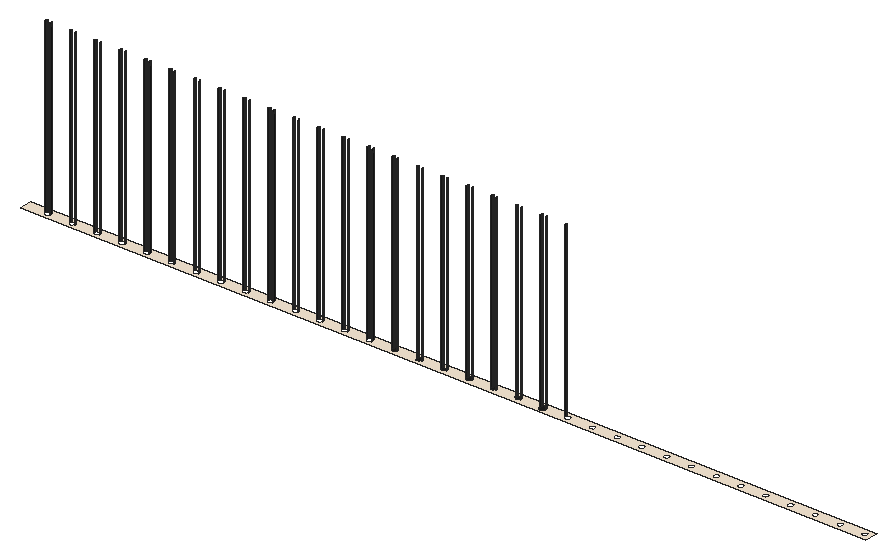
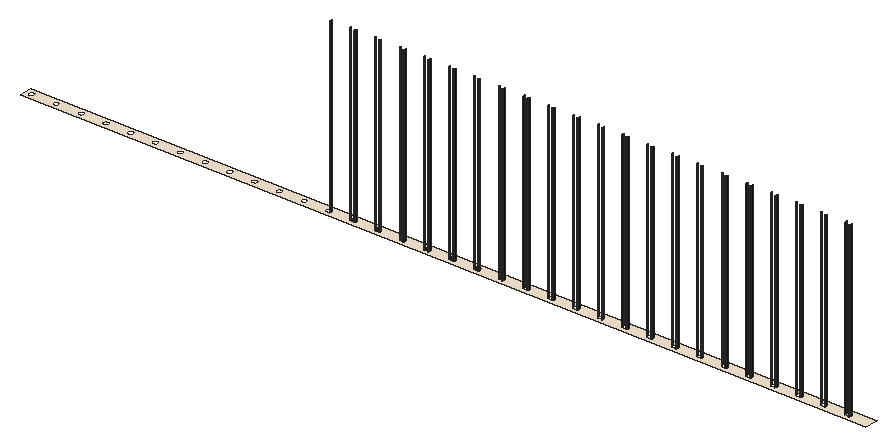
# SketchUp Ruby script. Lengths in inches.
U = 1.inch
M = Sketchup.active_model
def pt(a) = Geom::Point3d.new(a.map { |v| v * U })
def face(e, loops, mat)
  f = e.add_face(loops[0].map { |a| pt(a) })
  loops[1..].each { |l| e.add_face(l.map { |a| pt(a) }).erase! }
  f.material = f.back_material = mat if mat
  f
end
# faces: each face lists its corners as indices into pts; further lists are holes
def faces(e, pts, list, mat = nil) = list.each { |f| face(e, (f[0].is_a?(Array) ? f : [f]).map { |l| l.map { |i| pts[i] } }, mat) }
# xy, xz, yz: faces in a plane at the given z, y or x. An outline is a flat list of corners, or four numbers for a rectangle; further outlines are holes
def ring(l) = l.size == 4 ? [[l[0], l[1]], [l[2], l[1]], [l[2], l[3]], [l[0], l[3]]] : l.each_slice(2).to_a
def flat(e, list, mat, &to3) = list.each { |f| face(e, (f[0].is_a?(Array) ? f : [f]).map { |l| ring(l).map { |u, v| to3.(u, v) } }, mat) }
def xy(e, z, list, mat = nil) = flat(e, list, mat) { |x, y| [x, y, z] }
def xz(e, y, list, mat = nil) = flat(e, list, mat) { |x, z| [x, y, z] }
def yz(e, x, list, mat = nil) = flat(e, list, mat) { |y, z| [x, y, z] }
def lines(e, pts, list) = list.each { |a, b| e.add_line(pt(pts[a]), pt(pts[b])) }
# prism: a flat outline (further loops are holes) pulled along v
def prism(e, loops, v, mat = nil)
  f = face(e, loops, mat); d = Geom::Vector3d.new(v.map { |x| x * U })
  f.pushpull(f.normal.samedirection?(d) ? d.length : -d.length)
end
def box(e, o, s, mat = nil) = prism(e, [[o, [o[0] + s[0], o[1], o[2]], [o[0] + s[0], o[1] + s[1], o[2]], [o[0], o[1] + s[1], o[2]]]], [0, 0, s[2]], mat)
def at(x, y, z, deg = 0) = Geom::Transformation.translation(pt([x, y, z])) * Geom::Transformation.rotation(ORIGIN, Z_AXIS, deg.degrees)
def axes(o, x, y, z) = Geom::Transformation.new([*x, 0, *y, 0, *z, 0, *pt(o).to_a, 1])
def part(name) = M.definitions.add(name)
# library, detail: a bought-in or finely detailed component or shape, given as its bounding box
def library(name, o, s) = part(name).tap { |d| box(d.entities, o, s) }
def detail(e, o, s) = box(e.add_group.entities, o, s)
def put(e, d, t, mat = nil) = e.add_instance(d, t).tap { |i| i.material = mat if mat }
def group(e, t, mat = nil) = e.add_group.tap { |g| g.transformation = t; g.material = mat if mat }.entities
root = M.entities
M.materials.add("[0028_AntiqueWhite]").color = [250, 235, 215]
M.materials.add("[Color M08]").color = [30, 30, 30]
xy(root,177,[[[50.75,194.125,206.5625,196.4375],[54.79,194.68,54.65,194.71,54.52,194.79,54.42,194.89,54.35,195.02,54.31,195.16,54.31,195.31,54.34,195.45,54.42,195.58,54.52,195.68,54.65,195.75,54.79,195.79,54.9375,195.79,55.08,195.75,55.21,195.68,55.31,195.58,55.38,195.45,55.42,195.31,55.42,195.16,55.38,195.02,55.3125,194.89,55.21,194.79,55.08,194.72,54.9375,194.68],[59.35,194.68,59.21,194.71,59.09,194.79,58.98,194.89,58.91,195.02,58.87,195.16,58.87,195.31,58.91,195.45,58.98,195.58,59.08,195.68,59.21,195.75,59.35,195.79,59.5,195.79,59.64,195.75,59.77,195.68,59.87,195.58,59.95,195.45,59.98,195.31,59.99,195.16,59.95,195.02,59.875,194.89,59.77,194.79,59.64,194.72,59.5,194.68],[63.92,194.68,63.78,194.71,63.65,194.79,63.54,194.89,63.47,195.02,63.43,195.16,63.43,195.31,63.47,195.45,63.54,195.58,63.65,195.68,63.77,195.75,63.92,195.79,64.0625,195.79,64.2,195.75,64.33,195.68,64.44,195.58,64.51,195.45,64.55,195.31,64.55,195.16,64.51,195.02,64.4375,194.89,64.33,194.79,64.21,194.72,64.0625,194.68],[68.48,194.68,68.34,194.71,68.21,194.79,68.11,194.89,68.03,195.02,67.99,195.16,67.99,195.31,68.03,195.45,68.11,195.58,68.21,195.68,68.34,195.75,68.48,195.79,68.625,195.79,68.77,195.75,68.89,195.68,69,195.58,69.07,195.45,69.11,195.31,69.11,195.16,69.07,195.02,69,194.89,68.9,194.79,68.77,194.72,68.625,194.68],[73.04,194.68,72.9,194.71,72.77,194.79,72.67,194.89,72.6,195.02,72.56,195.16,72.56,195.31,72.59,195.45,72.67,195.58,72.77,195.68,72.9,195.75,73.04,195.79,73.1875,195.79,73.33,195.75,73.46,195.68,73.56,195.58,73.63,195.45,73.67,195.31,73.67,195.16,73.63,195.02,73.5625,194.89,73.46,194.79,73.33,194.72,73.1875,194.68],[77.6,194.68,77.46,194.71,77.34,194.79,77.23,194.89,77.16,195.02,77.12,195.16,77.12,195.31,77.16,195.45,77.23,195.58,77.33,195.68,77.46,195.75,77.6,195.79,77.75,195.79,77.89,195.75,78.02,195.68,78.12,195.58,78.2,195.45,78.23,195.31,78.24,195.16,78.2,195.02,78.125,194.89,78.02,194.79,77.89,194.72,77.75,194.68],[82.17,194.68,82.03,194.71,81.9,194.79,81.79,194.89,81.72,195.02,81.68,195.16,81.68,195.31,81.72,195.45,81.79,195.58,81.9,195.68,82.02,195.75,82.17,195.79,82.3125,195.79,82.45,195.75,82.58,195.68,82.69,195.58,82.76,195.45,82.8,195.31,82.8,195.16,82.76,195.02,82.6875,194.89,82.58,194.79,82.46,194.72,82.3125,194.68],[86.73,194.68,86.59,194.71,86.46,194.79,86.36,194.89,86.28,195.02,86.24,195.16,86.24,195.31,86.28,195.45,86.36,195.58,86.46,195.68,86.59,195.75,86.73,195.79,86.875,195.79,87.02,195.75,87.14,195.68,87.25,195.58,87.32,195.45,87.36,195.31,87.36,195.16,87.32,195.02,87.25,194.89,87.15,194.79,87.02,194.72,86.875,194.68],[91.29,194.68,91.15,194.71,91.02,194.79,90.92,194.89,90.85,195.02,90.81,195.16,90.81,195.31,90.84,195.45,90.92,195.58,91.02,195.68,91.15,195.75,91.29,195.79,91.4375,195.79,91.58,195.75,91.71,195.68,91.81,195.58,91.88,195.45,91.92,195.31,91.92,195.16,91.88,195.02,91.8125,194.89,91.71,194.79,91.58,194.72,91.4375,194.68],[95.85,194.68,95.71,194.71,95.59,194.79,95.48,194.89,95.41,195.02,95.37,195.16,95.37,195.31,95.41,195.45,95.48,195.58,95.58,195.68,95.71,195.75,95.85,195.79,96,195.79,96.14,195.75,96.27,195.68,96.37,195.58,96.45,195.45,96.48,195.31,96.49,195.16,96.45,195.02,96.375,194.89,96.27,194.79,96.14,194.72,96,194.68],[100.42,194.68,100.28,194.71,100.15,194.79,100.04,194.89,99.97,195.02,99.93,195.16,99.93,195.31,99.97,195.45,100.04,195.58,100.15,195.68,100.27,195.75,100.42,195.79,100.5625,195.79,100.7,195.75,100.83,195.68,100.94,195.58,101.01,195.45,101.05,195.31,101.05,195.16,101.01,195.02,100.9375,194.89,100.83,194.79,100.71,194.72,100.5625,194.68],[104.98,194.68,104.84,194.71,104.71,194.79,104.61,194.89,104.53,195.02,104.49,195.16,104.49,195.31,104.53,195.45,104.61,195.58,104.71,195.68,104.84,195.75,104.98,195.79,105.125,195.79,105.27,195.75,105.39,195.68,105.5,195.58,105.57,195.45,105.61,195.31,105.61,195.16,105.57,195.02,105.5,194.89,105.4,194.79,105.27,194.72,105.125,194.68],[109.54,194.68,109.4,194.71,109.27,194.79,109.17,194.89,109.1,195.02,109.06,195.16,109.06,195.31,109.09,195.45,109.17,195.58,109.27,195.68,109.4,195.75,109.54,195.79,109.6875,195.79,109.83,195.75,109.96,195.68,110.06,195.58,110.13,195.45,110.17,195.31,110.17,195.16,110.13,195.02,110.0625,194.89,109.96,194.79,109.83,194.72,109.6875,194.68],[114.1,194.68,113.96,194.71,113.84,194.79,113.73,194.89,113.66,195.02,113.62,195.16,113.62,195.31,113.66,195.45,113.73,195.58,113.83,195.68,113.96,195.75,114.1,195.79,114.25,195.79,114.39,195.75,114.52,195.68,114.62,195.58,114.7,195.45,114.73,195.31,114.74,195.16,114.7,195.02,114.625,194.89,114.52,194.79,114.39,194.72,114.25,194.68],[118.67,194.68,118.53,194.71,118.4,194.79,118.29,194.89,118.22,195.02,118.18,195.16,118.18,195.31,118.22,195.45,118.29,195.58,118.4,195.68,118.52,195.75,118.67,195.79,118.8125,195.79,118.95,195.75,119.08,195.68,119.19,195.58,119.26,195.45,119.3,195.31,119.3,195.16,119.26,195.02,119.1875,194.89,119.08,194.79,118.96,194.72,118.8125,194.68],[123.23,194.68,123.09,194.71,122.96,194.79,122.86,194.89,122.78,195.02,122.74,195.16,122.74,195.31,122.78,195.45,122.86,195.58,122.96,195.68,123.09,195.75,123.23,195.79,123.375,195.79,123.52,195.75,123.64,195.68,123.75,195.58,123.82,195.45,123.86,195.31,123.86,195.16,123.82,195.02,123.75,194.89,123.65,194.79,123.52,194.72,123.375,194.68],[127.79,194.68,127.65,194.71,127.52,194.79,127.42,194.89,127.35,195.02,127.31,195.16,127.31,195.31,127.34,195.45,127.42,195.58,127.52,195.68,127.65,195.75,127.79,195.79,127.9375,195.79,128.08,195.75,128.21,195.68,128.31,195.58,128.38,195.45,128.42,195.31,128.42,195.16,128.38,195.02,128.3125,194.89,128.21,194.79,128.08,194.72,127.9375,194.68],[132.35,194.68,132.21,194.71,132.09,194.79,131.98,194.89,131.91,195.02,131.87,195.16,131.87,195.31,131.91,195.45,131.98,195.58,132.08,195.68,132.21,195.75,132.35,195.79,132.5,195.79,132.64,195.75,132.77,195.68,132.87,195.58,132.95,195.45,132.98,195.31,132.99,195.16,132.95,195.02,132.875,194.89,132.77,194.79,132.64,194.72,132.5,194.68],[136.92,194.68,136.78,194.71,136.65,194.79,136.54,194.89,136.47,195.02,136.43,195.16,136.43,195.31,136.47,195.45,136.54,195.58,136.65,195.68,136.77,195.75,136.92,195.79,137.0625,195.79,137.2,195.75,137.33,195.68,137.44,195.58,137.51,195.45,137.55,195.31,137.55,195.16,137.51,195.02,137.4375,194.89,137.33,194.79,137.21,194.72,137.0625,194.68],[141.48,194.68,141.34,194.71,141.21,194.79,141.11,194.89,141.03,195.02,140.99,195.16,140.99,195.31,141.03,195.45,141.11,195.58,141.21,195.68,141.34,195.75,141.48,195.79,141.625,195.79,141.77,195.75,141.89,195.68,142,195.58,142.07,195.45,142.11,195.31,142.11,195.16,142.07,195.02,142,194.89,141.9,194.79,141.77,194.72,141.625,194.68],[146.04,194.68,145.9,194.71,145.77,194.79,145.67,194.89,145.6,195.02,145.56,195.16,145.56,195.31,145.59,195.45,145.67,195.58,145.77,195.68,145.9,195.75,146.04,195.79,146.1875,195.79,146.33,195.75,146.46,195.68,146.56,195.58,146.63,195.45,146.67,195.31,146.67,195.16,146.63,195.02,146.5625,194.89,146.46,194.79,146.33,194.72,146.1875,194.68],[150.6,194.68,150.46,194.71,150.34,194.79,150.23,194.89,150.16,195.02,150.12,195.16,150.12,195.31,150.16,195.45,150.23,195.58,150.33,195.68,150.46,195.75,150.6,195.79,150.75,195.79,150.89,195.75,151.02,195.68,151.12,195.58,151.2,195.45,151.23,195.31,151.24,195.16,151.2,195.02,151.125,194.89,151.02,194.79,150.89,194.72,150.75,194.68],[155.17,194.68,155.03,194.71,154.9,194.79,154.79,194.89,154.72,195.02,154.68,195.16,154.68,195.31,154.72,195.45,154.79,195.58,154.9,195.68,155.02,195.75,155.17,195.79,155.3125,195.79,155.45,195.75,155.58,195.68,155.69,195.58,155.76,195.45,155.8,195.31,155.8,195.16,155.76,195.02,155.6875,194.89,155.58,194.79,155.46,194.72,155.3125,194.68],[159.73,194.68,159.59,194.71,159.46,194.79,159.36,194.89,159.28,195.02,159.24,195.16,159.24,195.31,159.28,195.45,159.36,195.58,159.46,195.68,159.59,195.75,159.73,195.79,159.875,195.79,160.02,195.75,160.14,195.68,160.25,195.58,160.32,195.45,160.36,195.31,160.36,195.16,160.32,195.02,160.25,194.89,160.15,194.79,160.02,194.72,159.875,194.68],[164.29,194.68,164.15,194.71,164.02,194.79,163.92,194.89,163.85,195.02,163.81,195.16,163.81,195.31,163.84,195.45,163.92,195.58,164.02,195.68,164.15,195.75,164.29,195.79,164.4375,195.79,164.58,195.75,164.71,195.68,164.81,195.58,164.88,195.45,164.92,195.31,164.92,195.16,164.88,195.02,164.8125,194.89,164.71,194.79,164.58,194.72,164.4375,194.68],[168.85,194.68,168.71,194.71,168.59,194.79,168.48,194.89,168.41,195.02,168.37,195.16,168.37,195.31,168.41,195.45,168.48,195.58,168.58,195.68,168.71,195.75,168.85,195.79,169,195.79,169.14,195.75,169.27,195.68,169.37,195.58,169.45,195.45,169.48,195.31,169.49,195.16,169.45,195.02,169.375,194.89,169.27,194.79,169.14,194.72,169,194.68],[173.42,194.68,173.28,194.71,173.15,194.79,173.04,194.89,172.97,195.02,172.93,195.16,172.93,195.31,172.97,195.45,173.04,195.58,173.15,195.68,173.27,195.75,173.42,195.79,173.5625,195.79,173.7,195.75,173.83,195.68,173.94,195.58,174.01,195.45,174.05,195.31,174.05,195.16,174.01,195.02,173.9375,194.89,173.83,194.79,173.71,194.72,173.5625,194.68],[177.98,194.68,177.84,194.71,177.71,194.79,177.61,194.89,177.53,195.02,177.49,195.16,177.49,195.31,177.53,195.45,177.61,195.58,177.71,195.68,177.84,195.75,177.98,195.79,178.125,195.79,178.27,195.75,178.39,195.68,178.5,195.58,178.57,195.45,178.61,195.31,178.61,195.16,178.57,195.02,178.5,194.89,178.4,194.79,178.27,194.72,178.125,194.68],[182.54,194.68,182.4,194.71,182.27,194.79,182.17,194.89,182.1,195.02,182.06,195.16,182.06,195.31,182.09,195.45,182.17,195.58,182.27,195.68,182.4,195.75,182.54,195.79,182.6875,195.79,182.83,195.75,182.96,195.68,183.06,195.58,183.13,195.45,183.17,195.31,183.17,195.16,183.13,195.02,183.0625,194.89,182.96,194.79,182.83,194.72,182.6875,194.68],[187.1,194.68,186.96,194.71,186.84,194.79,186.73,194.89,186.66,195.02,186.62,195.16,186.62,195.31,186.66,195.45,186.73,195.58,186.83,195.68,186.96,195.75,187.1,195.79,187.25,195.79,187.39,195.75,187.52,195.68,187.62,195.58,187.7,195.45,187.73,195.31,187.74,195.16,187.7,195.02,187.625,194.89,187.52,194.79,187.39,194.72,187.25,194.68],[191.67,194.68,191.53,194.71,191.4,194.79,191.29,194.89,191.22,195.02,191.18,195.16,191.18,195.31,191.22,195.45,191.29,195.58,191.4,195.68,191.52,195.75,191.67,195.79,191.8125,195.79,191.95,195.75,192.08,195.68,192.19,195.58,192.26,195.45,192.3,195.31,192.3,195.16,192.26,195.02,192.1875,194.89,192.08,194.79,191.96,194.72,191.8125,194.68],[196.23,194.68,196.09,194.71,195.96,194.79,195.86,194.89,195.78,195.02,195.74,195.16,195.74,195.31,195.78,195.45,195.86,195.58,195.96,195.68,196.09,195.75,196.23,195.79,196.375,195.79,196.52,195.75,196.64,195.68,196.75,195.58,196.82,195.45,196.86,195.31,196.86,195.16,196.82,195.02,196.75,194.89,196.65,194.79,196.52,194.72,196.375,194.68],[200.79,194.68,200.65,194.71,200.52,194.79,200.42,194.89,200.35,195.02,200.31,195.16,200.31,195.31,200.34,195.45,200.42,195.58,200.52,195.68,200.65,195.75,200.79,195.79,200.9375,195.79,201.08,195.75,201.21,195.68,201.31,195.58,201.38,195.45,201.42,195.31,201.42,195.16,201.38,195.02,201.3125,194.89,201.21,194.79,201.08,194.72,200.9375,194.68],[205.35,194.68,205.21,194.71,205.09,194.79,204.98,194.89,204.91,195.02,204.87,195.16,204.87,195.31,204.91,195.45,204.98,195.58,205.08,195.68,205.21,195.75,205.35,195.79,205.5,195.79,205.64,195.75,205.77,195.68,205.87,195.58,205.95,195.45,205.98,195.31,205.99,195.16,205.95,195.02,205.875,194.89,205.77,194.79,205.64,194.72,205.5,194.68]]],"[0028_AntiqueWhite]")
xy(root,177,[[118.67,194.68,118.53,194.71,118.4,194.79,118.29,194.89,118.22,195.02,118.18,195.16,118.18,195.31,118.22,195.45,118.29,195.58,118.4,195.68,118.52,195.75,118.67,195.79,118.8125,195.79,118.95,195.75,119.08,195.68,119.19,195.58,119.26,195.45,119.3,195.31,119.3,195.16,119.26,195.02,119.1875,194.89,119.08,194.79,118.96,194.72,118.8125,194.68],[123.23,194.68,123.09,194.71,122.96,194.79,122.86,194.89,122.78,195.02,122.74,195.16,122.74,195.31,122.78,195.45,122.86,195.58,122.96,195.68,123.09,195.75,123.23,195.79,123.375,195.79,123.52,195.75,123.64,195.68,123.75,195.58,123.82,195.45,123.86,195.31,123.86,195.16,123.82,195.02,123.75,194.89,123.65,194.79,123.52,194.72,123.375,194.68],[127.79,194.68,127.65,194.71,127.52,194.79,127.42,194.89,127.35,195.02,127.31,195.16,127.31,195.31,127.34,195.45,127.42,195.58,127.52,195.68,127.65,195.75,127.79,195.79,127.9375,195.79,128.08,195.75,128.21,195.68,128.31,195.58,128.38,195.45,128.42,195.31,128.42,195.16,128.38,195.02,128.3125,194.89,128.21,194.79,128.08,194.72,127.9375,194.68],[132.35,194.68,132.21,194.71,132.09,194.79,131.98,194.89,131.91,195.02,131.87,195.16,131.87,195.31,131.91,195.45,131.98,195.58,132.08,195.68,132.21,195.75,132.35,195.79,132.5,195.79,132.64,195.75,132.77,195.68,132.87,195.58,132.95,195.45,132.98,195.31,132.99,195.16,132.95,195.02,132.875,194.89,132.77,194.79,132.64,194.72,132.5,194.68],[136.92,194.68,136.78,194.71,136.65,194.79,136.54,194.89,136.47,195.02,136.43,195.16,136.43,195.31,136.47,195.45,136.54,195.58,136.65,195.68,136.77,195.75,136.92,195.79,137.0625,195.79,137.2,195.75,137.33,195.68,137.44,195.58,137.51,195.45,137.55,195.31,137.55,195.16,137.51,195.02,137.4375,194.89,137.33,194.79,137.21,194.72,137.0625,194.68],
  [141.48,194.68,141.34,194.71,141.21,194.79,141.11,194.89,141.03,195.02,140.99,195.16,140.99,195.31,141.03,195.45,141.11,195.58,141.21,195.68,141.34,195.75,141.48,195.79,141.625,195.79,141.77,195.75,141.89,195.68,142,195.58,142.07,195.45,142.11,195.31,142.11,195.16,142.07,195.02,142,194.89,141.9,194.79,141.77,194.72,141.625,194.68],[146.04,194.68,145.9,194.71,145.77,194.79,145.67,194.89,145.6,195.02,145.56,195.16,145.56,195.31,145.59,195.45,145.67,195.58,145.77,195.68,145.9,195.75,146.04,195.79,146.1875,195.79,146.33,195.75,146.46,195.68,146.56,195.58,146.63,195.45,146.67,195.31,146.67,195.16,146.63,195.02,146.5625,194.89,146.46,194.79,146.33,194.72,146.1875,194.68]],"[Color M08]")
yz(root,55.42,[[195.16,177,195.31,208.66]],"[Color M08]")
yz(root,64.55,[[195.16,177,195.31,208.66]],"[Color M08]")
yz(root,69.11,[[195.16,177,195.31,208.66]],"[Color M08]")
yz(root,73.67,[[195.16,177,195.31,208.66]],"[Color M08]")
yz(root,82.8,[[195.16,177,195.31,208.66]],"[Color M08]")
yz(root,87.36,[[195.16,177,195.31,208.66]],"[Color M08]")
yz(root,91.92,[[195.16,177,195.31,208.66]],"[Color M08]")
yz(root,101.05,[[195.16,177,195.31,208.66]],"[Color M08]")
yz(root,105.61,[[195.16,177,195.31,208.66]],"[Color M08]")
yz(root,110.17,[[195.16,177,195.31,208.66]],"[Color M08]")
yz(root,119.3,[[195.16,177,195.31,208.66]],"[Color M08]")
yz(root,123.86,[[195.16,177,195.31,208.66]],"[Color M08]")
yz(root,128.42,[[195.16,177,195.31,208.66]],"[Color M08]")
yz(root,137.55,[[195.16,177,195.31,208.66]],"[Color M08]")
yz(root,142.11,[[195.16,177,195.31,208.66]],"[Color M08]")
yz(root,146.67,[[195.16,177,195.31,208.66]],"[Color M08]")
p = [[59.99,195.16,177],[59.98,195.31,177],[59.98,195.31,208.66],[59.99,195.16,208.66],[78.24,195.16,177],[78.23,195.31,177],
  [78.23,195.31,208.66],[78.24,195.16,208.66],[96.49,195.16,177],[96.48,195.31,177],[96.48,195.31,208.66],[96.49,195.16,208.66],
  [114.74,195.16,177],[114.73,195.31,177],[114.73,195.31,208.66],[114.74,195.16,208.66],[132.99,195.16,177],[132.98,195.31,177],
  [132.98,195.31,208.66],[132.99,195.16,208.66],[54.34,195.45,177],[54.31,195.31,177],[54.31,195.31,208.66],[54.34,195.45,208.66],
  [55.42,195.31,177],[55.38,195.45,177],[55.38,195.45,208.66],[55.42,195.31,208.66],[58.91,195.45,177],[58.87,195.31,177],
  [58.87,195.31,208.66],[58.91,195.45,208.66],[59.95,195.45,177],[59.95,195.45,208.66],[63.47,195.45,177],[63.43,195.31,177],
  [63.43,195.31,208.66],[63.47,195.45,208.66],[64.55,195.31,177],[64.51,195.45,177],[64.51,195.45,208.66],[64.55,195.31,208.66],
  [68.03,195.45,177],[67.99,195.31,177],[67.99,195.31,208.66],[68.03,195.45,208.66],[69.11,195.31,177],[69.07,195.45,177],
  [69.07,195.45,208.66],[69.11,195.31,208.66],[72.59,195.45,177],[72.56,195.31,177],[72.56,195.31,208.66],[72.59,195.45,208.66],
  [73.67,195.31,177],[73.63,195.45,177],[73.63,195.45,208.66],[73.67,195.31,208.66],[77.16,195.45,177],[77.12,195.31,177],
  [77.12,195.31,208.66],[77.16,195.45,208.66],[78.2,195.45,177],[78.2,195.45,208.66],[81.72,195.45,177],[81.68,195.31,177],
  [81.68,195.31,208.66],[81.72,195.45,208.66],[82.8,195.31,177],[82.76,195.45,177],[82.76,195.45,208.66],[82.8,195.31,208.66],
  [86.28,195.45,177],[86.24,195.31,177],[86.24,195.31,208.66],[86.28,195.45,208.66],[87.36,195.31,177],[87.32,195.45,177],
  [87.32,195.45,208.66],[87.36,195.31,208.66],[90.84,195.45,177],[90.81,195.31,177],[90.81,195.31,208.66],[90.84,195.45,208.66],
  [91.92,195.31,177],[91.88,195.45,177],[91.88,195.45,208.66],[91.92,195.31,208.66],[95.41,195.45,177],[95.37,195.31,177],
  [95.37,195.31,208.66],[95.41,195.45,208.66],[96.45,195.45,177],[96.45,195.45,208.66],[99.97,195.45,177],[99.93,195.31,177],
  [99.93,195.31,208.66],[99.97,195.45,208.66],[101.05,195.31,177],[101.01,195.45,177],[101.01,195.45,208.66],[101.05,195.31,208.66],
  [104.53,195.45,177],[104.49,195.31,177],[104.49,195.31,208.66],[104.53,195.45,208.66],[105.61,195.31,177],[105.57,195.45,177],
  [105.57,195.45,208.66],[105.61,195.31,208.66],[109.09,195.45,177],[109.06,195.31,177],[109.06,195.31,208.66],[109.09,195.45,208.66],
  [110.17,195.31,177],[110.13,195.45,177],[110.13,195.45,208.66],[110.17,195.31,208.66],[113.66,195.45,177],[113.62,195.31,177],
  [113.62,195.31,208.66],[113.66,195.45,208.66],[114.7,195.45,177],[114.7,195.45,208.66],[118.22,195.45,177],[118.18,195.31,177],
  [118.18,195.31,208.66],[118.22,195.45,208.66],[119.3,195.31,177],[119.26,195.45,177],[119.26,195.45,208.66],[119.3,195.31,208.66],
  [122.78,195.45,177],[122.74,195.31,177],[122.74,195.31,208.66],[122.78,195.45,208.66],[123.86,195.31,177],[123.82,195.45,177],
  [123.82,195.45,208.66],[123.86,195.31,208.66],[127.34,195.45,177],[127.31,195.31,177],[127.31,195.31,208.66],[127.34,195.45,208.66],
  [128.42,195.31,177],[128.38,195.45,177],[128.38,195.45,208.66],[128.42,195.31,208.66],[131.91,195.45,177],[131.87,195.31,177],
  [131.87,195.31,208.66],[131.91,195.45,208.66],[132.95,195.45,177],[132.95,195.45,208.66],[136.47,195.45,177],[136.43,195.31,177],
  [136.43,195.31,208.66],[136.47,195.45,208.66],[137.55,195.31,177],[137.51,195.45,177],[137.51,195.45,208.66],[137.55,195.31,208.66],
  [141.03,195.45,177],[140.99,195.31,177],[140.99,195.31,208.66],[141.03,195.45,208.66],[142.11,195.31,177],[142.07,195.45,177],
  [142.07,195.45,208.66],[142.11,195.31,208.66],[145.59,195.45,177],[145.56,195.31,177],[145.56,195.31,208.66],[145.59,195.45,208.66],
  [146.67,195.31,177],[146.63,195.45,177],[146.63,195.45,208.66],[146.67,195.31,208.66],[150.16,195.45,177],[150.12,195.31,177],
  [150.12,195.31,208.66],[150.16,195.45,208.66],[54.42,195.58,177],[54.42,195.58,208.66],[58.98,195.58,177],[58.98,195.58,208.66],
  [63.54,195.58,177],[63.54,195.58,208.66],[68.11,195.58,177],[68.11,195.58,208.66],[72.67,195.58,177],[72.67,195.58,208.66],
  [77.23,195.58,177],[77.23,195.58,208.66],[81.79,195.58,177],[81.79,195.58,208.66],[86.36,195.58,177],[86.36,195.58,208.66],
  [90.92,195.58,177],[90.92,195.58,208.66],[95.48,195.58,177],[95.48,195.58,208.66],[100.04,195.58,177],[100.04,195.58,208.66],
  [104.61,195.58,177],[104.61,195.58,208.66],[109.17,195.58,177],[109.17,195.58,208.66],[113.73,195.58,177],[113.73,195.58,208.66],
  [118.29,195.58,177],[118.29,195.58,208.66],[122.86,195.58,177],[122.86,195.58,208.66],[127.42,195.58,177],[127.42,195.58,208.66],
  [131.98,195.58,177],[131.98,195.58,208.66],[136.54,195.58,177],[136.54,195.58,208.66],[141.11,195.58,177],[141.11,195.58,208.66],
  [145.67,195.58,177],[145.67,195.58,208.66],[150.23,195.58,177],[150.23,195.58,208.66],[55.31,195.58,177],[55.31,195.58,208.66],
  [59.87,195.58,177],[59.87,195.58,208.66],[64.44,195.58,177],[64.44,195.58,208.66],[69,195.58,177],[69,195.58,208.66],
  [73.56,195.58,177],[73.56,195.58,208.66],[78.12,195.58,177],[78.12,195.58,208.66],[82.69,195.58,177],[82.69,195.58,208.66],
  [87.25,195.58,177],[87.25,195.58,208.66],[91.81,195.58,177],[91.81,195.58,208.66],[96.37,195.58,177],[96.37,195.58,208.66],
  [100.94,195.58,177],[100.94,195.58,208.66],[105.5,195.58,177],[105.5,195.58,208.66],[110.06,195.58,177],[110.06,195.58,208.66],
  [114.62,195.58,177],[114.62,195.58,208.66],[119.19,195.58,177],[119.19,195.58,208.66],[123.75,195.58,177],[123.75,195.58,208.66],
  [128.31,195.58,177],[128.31,195.58,208.66],[132.87,195.58,177],[132.87,195.58,208.66],[137.44,195.58,177],[137.44,195.58,208.66],
  [142,195.58,177],[142,195.58,208.66],[146.56,195.58,177],[146.56,195.58,208.66],[54.52,195.68,177],[54.52,195.68,208.66],
  [59.08,195.68,177],[59.08,195.68,208.66],[63.65,195.68,177],[63.65,195.68,208.66],[68.21,195.68,177],[68.21,195.68,208.66],
  [72.77,195.68,177],[72.77,195.68,208.66],[77.33,195.68,177],[77.33,195.68,208.66],[81.9,195.68,177],[81.9,195.68,208.66],
  [86.46,195.68,177],[86.46,195.68,208.66],[91.02,195.68,177],[91.02,195.68,208.66],[95.58,195.68,177],[95.58,195.68,208.66],
  [100.15,195.68,177],[100.15,195.68,208.66],[104.71,195.68,177],[104.71,195.68,208.66],[109.27,195.68,177],[109.27,195.68,208.66],
  [113.83,195.68,177],[113.83,195.68,208.66],[118.4,195.68,177],[118.4,195.68,208.66],[122.96,195.68,177],[122.96,195.68,208.66],
  [127.52,195.68,177],[127.52,195.68,208.66],[132.08,195.68,177],[132.08,195.68,208.66],[136.65,195.68,177],[136.65,195.68,208.66],
  [141.21,195.68,177],[141.21,195.68,208.66],[145.77,195.68,177],[145.77,195.68,208.66]]
faces(root,p,[[0,1,2,3],[4,5,6,7],[8,9,10,11],[12,13,14,15],[16,17,18,19],[20,21,22,23],[24,25,26,27],[28,29,30,31],
  [1,32,33,2],[34,35,36,37],[38,39,40,41],[42,43,44,45],[46,47,48,49],[50,51,52,53],[54,55,56,57],[58,59,60,61],
  [5,62,63,6],[64,65,66,67],[68,69,70,71],[72,73,74,75],[76,77,78,79],[80,81,82,83],[84,85,86,87],[88,89,90,91],
  [9,92,93,10],[94,95,96,97],[98,99,100,101],[102,103,104,105],[106,107,108,109],[110,111,112,113],[114,115,116,117],[118,119,120,121],
  [13,122,123,14],[124,125,126,127],[128,129,130,131],[132,133,134,135],[136,137,138,139],[140,141,142,143],[144,145,146,147],[148,149,150,151],
  [17,152,153,18],[154,155,156,157],[158,159,160,161],[162,163,164,165],[166,167,168,169],[170,171,172,173],[174,175,176,177],[178,179,180,181],
  [182,20,23,183],[184,28,31,185],[186,34,37,187],[188,42,45,189],[190,50,53,191],[192,58,61,193],[194,64,67,195],[196,72,75,197],
  [198,80,83,199],[200,88,91,201],[202,94,97,203],[204,102,105,205],[206,110,113,207],[208,118,121,209],[210,124,127,211],[212,132,135,213],
  [214,140,143,215],[216,148,151,217],[218,154,157,219],[220,162,165,221],[222,170,173,223],[224,178,181,225],[25,226,227,26],[32,228,229,33],
  [39,230,231,40],[47,232,233,48],[55,234,235,56],[62,236,237,63],[69,238,239,70],[77,240,241,78],[85,242,243,86],[92,244,245,93],
  [99,246,247,100],[107,248,249,108],[115,250,251,116],[122,252,253,123],[129,254,255,130],[137,256,257,138],[145,258,259,146],[152,260,261,153],
  [159,262,263,160],[167,264,265,168],[175,266,267,176],[268,182,183,269],[270,184,185,271],[272,186,187,273],[274,188,189,275],[276,190,191,277],
  [278,192,193,279],[280,194,195,281],[282,196,197,283],[284,198,199,285],[286,200,201,287],[288,202,203,289],[290,204,205,291],[292,206,207,293],
  [294,208,209,295],[296,210,211,297],[298,212,213,299],[300,214,215,301],[302,216,217,303],[304,218,219,305],[306,220,221,307],[308,222,223,309]],"[Color M08]")
